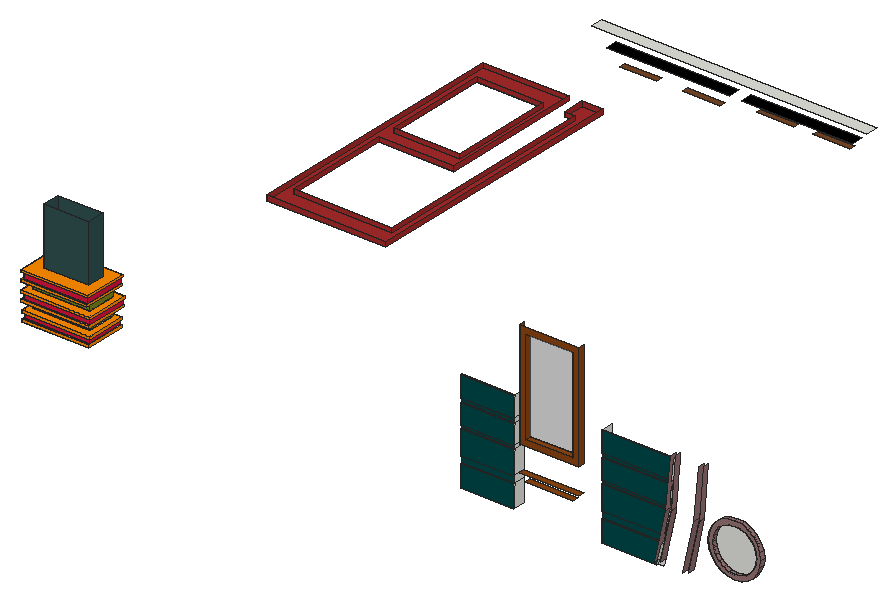
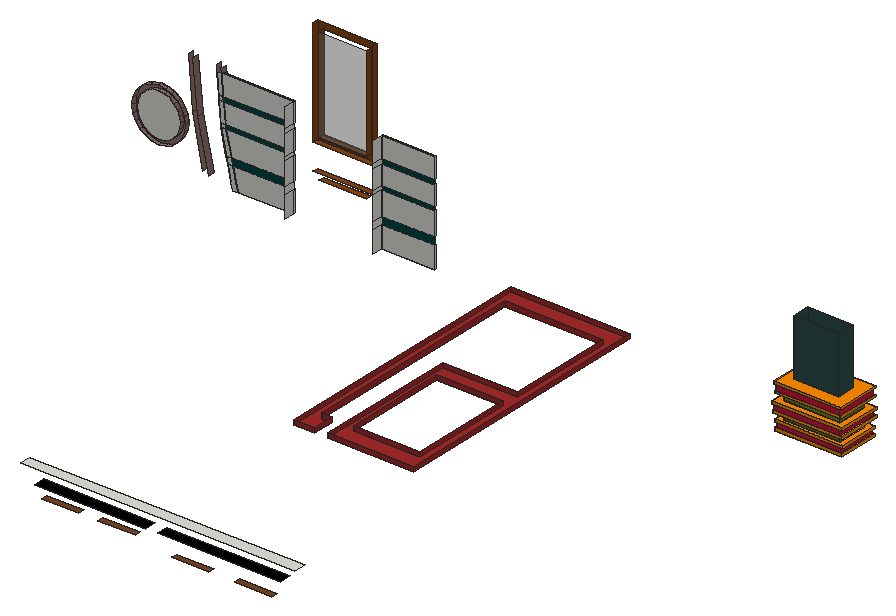
# SketchUp Ruby script. Lengths in inches.
U = 1.inch
M = Sketchup.active_model
def pt(a) = Geom::Point3d.new(a.map { |v| v * U })
def face(e, loops, mat)
  f = e.add_face(loops[0].map { |a| pt(a) })
  loops[1..].each { |l| e.add_face(l.map { |a| pt(a) }).erase! }
  f.material = f.back_material = mat if mat
  f
end
# faces: each face lists its corners as indices into pts; further lists are holes
def faces(e, pts, list, mat = nil) = list.each { |f| face(e, (f[0].is_a?(Array) ? f : [f]).map { |l| l.map { |i| pts[i] } }, mat) }
# xy, xz, yz: faces in a plane at the given z, y or x. An outline is a flat list of corners, or four numbers for a rectangle; further outlines are holes
def ring(l) = l.size == 4 ? [[l[0], l[1]], [l[2], l[1]], [l[2], l[3]], [l[0], l[3]]] : l.each_slice(2).to_a
def flat(e, list, mat, &to3) = list.each { |f| face(e, (f[0].is_a?(Array) ? f : [f]).map { |l| ring(l).map { |u, v| to3.(u, v) } }, mat) }
def xy(e, z, list, mat = nil) = flat(e, list, mat) { |x, y| [x, y, z] }
def xz(e, y, list, mat = nil) = flat(e, list, mat) { |x, z| [x, y, z] }
def yz(e, x, list, mat = nil) = flat(e, list, mat) { |y, z| [x, y, z] }
def lines(e, pts, list) = list.each { |a, b| e.add_line(pt(pts[a]), pt(pts[b])) }
# prism: a flat outline (further loops are holes) pulled along v
def prism(e, loops, v, mat = nil)
  f = face(e, loops, mat); d = Geom::Vector3d.new(v.map { |x| x * U })
  f.pushpull(f.normal.samedirection?(d) ? d.length : -d.length)
end
def box(e, o, s, mat = nil) = prism(e, [[o, [o[0] + s[0], o[1], o[2]], [o[0] + s[0], o[1] + s[1], o[2]], [o[0], o[1] + s[1], o[2]]]], [0, 0, s[2]], mat)
def at(x, y, z, deg = 0) = Geom::Transformation.translation(pt([x, y, z])) * Geom::Transformation.rotation(ORIGIN, Z_AXIS, deg.degrees)
def axes(o, x, y, z) = Geom::Transformation.new([*x, 0, *y, 0, *z, 0, *pt(o).to_a, 1])
def part(name) = M.definitions.add(name)
# library, detail: a bought-in or finely detailed component or shape, given as its bounding box
def library(name, o, s) = part(name).tap { |d| box(d.entities, o, s) }
def detail(e, o, s) = box(e.add_group.entities, o, s)
def put(e, d, t, mat = nil) = e.add_instance(d, t).tap { |i| i.material = mat if mat }
def group(e, t, mat = nil) = e.add_group.tap { |g| g.transformation = t; g.material = mat if mat }.entities
root = M.entities
M.materials.add("[0018_Brown]").color = [165, 42, 42]
M.materials.add("[0019_Crimson]").color = [220, 20, 60]
M.materials.add("[0039_DarkOrange]").color = [255, 140, 0]
M.materials.add("[0043_SaddleBrown]").color = [139, 69, 19]
M.materials.add("[0057_DarkKhaki]").color = [122, 132, 27]
M.materials.add("[0078_DarkSlateGray]").color = [47, 79, 79]
M.materials.add("[0119_RosyBrown]").color = [150, 114, 114]
M.materials.add("[0137_Black]").color = [0, 0, 0]
M.materials.add("[Color H08]").color = [0, 71, 71]
M.materials.add("[Translucent Glass Gray]").color = [128, 128, 128]
M.materials["[Translucent Glass Gray]"].alpha = 0.5
M.materials.add("[Wood Veneer 01]").color = [120, 70, 37]
xy(root,193.52,[[[1.625,647.11,35.57,667.86],[4,651.11,32.57,666.11]]],"[0039_DarkOrange]")
xy(root,194,[[221.0625,650.11,247.97,651.11],[292.45,650.11,320.32,651.11]],"[Color H08]")
xy(root,194.96,[[1.625,647.11,2.4375,648.11]])
xy(root,194.96,[[2.4375,647.11,35.57,647.11,35.57,667.86,1.625,667.86,1.625,648.11,2.4375,648.11,2.4375,667.36,35.13,667.36,35.13,648.11,2.4375,648.11]],"[0039_DarkOrange]")
xy(root,197.25,[[[1.3125,647.11,35.69,667.68],[2.4375,648.11,35.13,667.36]]],"[0039_DarkOrange]")
xy(root,198.71,[[[1.3125,647.11,35.69,667.68],[4,651.11,32.57,666.11]]],"[0039_DarkOrange]")
xy(root,202.27,[[[0.75,647.11,35.57,669.24],[4,651.11,32.57,666.11]]],"[0039_DarkOrange]")
xy(root,203.52,[[[0.75,647.11,35.57,669.24],[1.625,648.11,35.19,668.8]]],"[0039_DarkOrange]")
xy(root,204.94,[[221.0625,650.11,247.97,651.11],[292.45,650.11,323.1,651.11]],"[Color H08]")
xy(root,206.2,[[[0.75,647.11,36,669.24],[1.625,648.11,35.19,668.8]]],"[0039_DarkOrange]")
xy(root,207.46,[[[0.75,647.11,36,669.24],[4,651.11,32.57,666.11]]],"[0039_DarkOrange]")
xy(root,208.59,[[221.0625,650.11,247.97,651.11],[292.45,650.11,323.92,651.11]],"[Color H08]")
xy(root,211.52,[[[1.25,647.11,34.375,669.18],[1.625,648.11,34.13,668.8]]],"[0039_DarkOrange]")
xy(root,211.58,[[[1.625,648.11,34.13,668.8],[4,651.11,32.57,666.11]]],"[0039_DarkOrange]")
xy(root,211.75,[[258.01,645.11,281.88,648.11]],"[0043_SaddleBrown]")
xy(root,212.58,[[1.25,647.11,34.375,647.11,34.375,648.11,1.625,648.11,1.625,668.8,34.13,668.8,34.13,648.11,34.375,648.11,34.375,669.18,1.25,669.18]],"[0039_DarkOrange]")
xy(root,214.75,[[255.01,645.11,284.88,648.11]],"[0043_SaddleBrown]")
xy(root,215.72,[[[0.8125,647.11,34.75,669.36],[1.625,648.11,34.13,668.8]]],"[0039_DarkOrange]")
xy(root,215.75,[[82.37,924.36,101.18,927.36],[114.12,924.36,132.93,927.36]],"[Wood Veneer 01]")
xy(root,216.77,[[7,654.11,29.57,663.11]])
xy(root,216.77,[[[0.8125,647.11,34.75,669.36],[7,654.11,29.57,663.11]]],"[0039_DarkOrange]")
xy(root,219.3125,[[151.49,924.36,170.3,927.36],[179.93,924.36,198.74,927.36]],"[Wood Veneer 01]")
xy(root,220.65,[[221.0625,650.11,247.97,651.11],[292.45,650.11,326.64,651.11]],"[Color H08]")
xy(root,222.41,[[221.0625,650.11,247.97,651.11],[292.45,650.11,326.91,651.11]],"[Color H08]")
xy(root,224.07,[[78.125,921.36,140.28,927.36],[146.28,921.36,202.43,927.36]],"[0137_Black]")
xy(root,227.93,[[255.01,645.11,284.88,648.11]],"[0043_SaddleBrown]")
xy(root,230.93,[[258.01,645.11,281.88,648.11]],"[0043_SaddleBrown]")
xy(root,231.39,[[70.81,921.36,209.75,927.36]])
xy(root,232.54,[[221.0625,650.11,247.97,651.11],[292.45,650.11,327.84,651.11]],"[Color H08]")
xy(root,234.84,[[221.0625,650.11,247.97,651.11],[292.45,650.11,328.05,651.11]],"[Color H08]")
xy(root,243.17,[[[71.2,714.73,71.2,851.92,114.56,851.92,114.56,779.39,76.53,779.39,76.53,725.47,126.31,725.47,126.31,841.18,121.29,841.18,121.29,851.92,131.64,851.92,131.64,714.73],[76.53,788.7,109.94,841.18]]],"[0018_Brown]")
xz(root,645.11,[[[255.01,227.93,284.88,281.93],[258.01,230.93,281.88,278.93]]],"[0043_SaddleBrown]")
xz(root,647.11,[[1.625,193.52,35.57,194.96],[1.3125,197.25,35.69,198.71],[0.75,202.27,35.57,203.52],[0.75,206.2,36,207.46],[1.25,211.52,34.375,212.58],
  [0.8125,215.72,34.75,216.77]],"[0039_DarkOrange]")
xz(root,648.11,[[1.625,211.52,34.13,211.54],[1.625,211.54,34.13,211.58],[1.625,211.58,34.13,212.58]])
xz(root,648.11,[[2.4375,194.96,35.13,197.25],[1.625,203.52,35.19,206.2],[1.625,212.58,34.13,215.72]],"[0019_Crimson]")
xz(root,648.11,[[258.01,230.93,281.88,278.93]],"[Translucent Glass Gray]")
xz(root,649.11,[[[360.63,201.66,364.12,202.12,367.36,203.46,370.15,205.6,372.29,208.39,373.63,211.63,374.09,215.11,373.63,218.6,372.29,221.84,370.15,224.63,367.36,226.76,364.12,228.11,360.63,228.57,357.15,228.11,353.91,226.76,351.12,224.63,348.98,221.84,347.64,218.6,347.18,215.11,347.64,211.63,348.98,208.39,351.12,205.6,353.91,203.46,357.15,202.12],[360.63,204.07,357.78,204.45,355.11,205.55,352.83,207.31,351.07,209.59,349.97,212.26,349.59,215.11,349.97,217.97,351.07,220.64,352.83,222.92,355.11,224.68,357.78,225.78,360.63,226.16,363.49,225.78,366.16,224.68,368.44,222.92,370.2,220.64,371.3,217.97,371.68,215.11,371.3,212.26,370.2,209.59,368.44,207.31,366.16,205.55,363.49,204.45]]],"[0119_RosyBrown]")
xz(root,650.11,[[221.0625,194,247.97,204.94],[292.45,194,320.32,194,321.14,196.24,323.1,204.94,292.45,204.94],[221.0625,208.59,247.97,220.65],[292.45,208.59,323.92,208.59,326.64,220.65,292.45,220.65],[221.0625,222.41,247.97,232.54],
  [292.45,222.41,326.91,222.41,327.84,232.54,292.45,232.54],[221.0625,234.84,247.97,245.03],[292.45,234.84,328.05,234.84,328.99,245.03,292.45,245.03]],"[Color H08]")
xz(root,651.11,[[4,193.52,32.57,198.71],[221.0625,194,247.97,204.94],[292.45,194,292.45,204.94,323.1,204.94,321.14,196.24,320.32,194],[320.32,194,323.04,194,324.26,197.49,325.82,204.94,323.1,204.94,321.14,196.24],[4,202.27,32.57,207.46],
  [360.63,204.07,363.49,204.45,366.16,205.55,368.44,207.31,370.2,209.59,371.3,212.26,371.68,215.11,371.3,217.97,370.2,220.64,368.44,222.92,366.16,224.68,363.49,225.78,360.63,226.16,357.78,225.78,355.11,224.68,352.83,222.92,351.07,220.64,349.97,217.97,349.59,215.11,349.97,212.26,351.07,209.59,352.83,207.31,355.11,205.55,357.78,204.45],[323.1,204.94,325.82,204.94,326.59,208.59,323.92,208.59],[221.0625,208.59,247.97,220.65],[292.45,208.59,292.45,220.65,326.64,220.65,323.92,208.59],[323.92,208.59,326.59,208.59,329.12,220.65,326.64,220.65],
  [326.64,220.65,329.12,220.65,329.49,222.41,326.91,222.41,326.83,221.48],[221.0625,222.41,247.97,232.54],[292.45,222.41,292.45,232.54,327.84,232.54,326.91,222.41],[326.91,222.41,329.49,222.41,329.52,222.56,330.31,232.54,327.84,232.54],[327.84,232.54,330.31,232.54,330.49,234.84,328.05,234.84],
  [221.0625,234.84,247.97,245.03],[292.45,234.84,292.45,245.03,328.99,245.03,328.05,234.84],[328.05,234.84,330.49,234.84,331.29,245.03,328.99,245.03]])
xz(root,651.11,[[4,198.71,32.57,202.27],[4,207.46,32.57,211.58]],"[0057_DarkKhaki]")
xz(root,651.11,[[221.0625,204.94,247.97,208.59],[292.45,204.94,323.1,204.94,323.92,208.59,292.45,208.59],[221.0625,220.65,247.97,222.41],[292.45,220.65,326.64,220.65,326.83,221.48,326.91,222.41,292.45,222.41],[221.0625,232.54,247.97,234.84],
  [292.45,232.54,327.84,232.54,328.05,234.84,292.45,234.84]],"[Color H08]")
xz(root,654.11,[[7,216.77,29.57,245.51]],"[0078_DarkSlateGray]")
xz(root,663.11,[[7,216.77,29.57,245.51]],"[0078_DarkSlateGray]")
xz(root,666.11,[[4,193.52,32.57,198.71],[4,202.27,32.57,207.46]])
xz(root,666.11,[[4,198.71,32.57,202.27],[4,207.46,32.57,211.58]],"[0057_DarkKhaki]")
xz(root,667.36,[[2.4375,194.96,35.13,197.25]],"[0019_Crimson]")
xz(root,667.68,[[1.3125,197.25,35.69,198.71]],"[0039_DarkOrange]")
xz(root,667.86,[[1.625,193.52,35.57,194.96]],"[0039_DarkOrange]")
xz(root,668.8,[[1.625,211.52,34.13,211.58],[1.625,211.58,34.13,212.58]])
xz(root,668.8,[[1.625,203.52,35.19,206.2],[1.625,212.58,34.13,215.72]],"[0019_Crimson]")
xz(root,669.18,[[1.25,211.52,34.375,212.58]],"[0039_DarkOrange]")
xz(root,669.24,[[0.75,202.27,35.57,203.52],[0.75,206.2,36,207.46]],"[0039_DarkOrange]")
xz(root,669.36,[[0.8125,215.72,34.75,216.77]],"[0039_DarkOrange]")
xz(root,714.73,[[71.2,243.17,131.64,245.51]],"[0018_Brown]")
xz(root,725.47,[[76.53,243.17,126.31,245.51]],"[0018_Brown]")
xz(root,779.39,[[76.53,243.17,114.56,245.51]],"[0018_Brown]")
xz(root,788.7,[[76.53,243.17,109.94,245.51]],"[0018_Brown]")
xz(root,841.18,[[76.53,243.17,109.94,245.51],[121.29,243.17,126.31,245.51]],"[0018_Brown]")
xz(root,851.92,[[71.2,243.17,114.56,245.51],[121.29,243.17,131.64,245.51]],"[0018_Brown]")
yz(root,0.75,[[647.11,202.27,669.24,203.52],[647.11,206.2,669.24,207.46]],"[0039_DarkOrange]")
yz(root,0.8125,[[647.11,215.72,669.36,216.77]],"[0039_DarkOrange]")
yz(root,1.25,[[647.11,211.52,669.18,212.58]],"[0039_DarkOrange]")
yz(root,1.3125,[[647.11,197.25,667.68,198.71]],"[0039_DarkOrange]")
yz(root,1.625,[[648.11,211.52,668.8,211.58],[648.11,211.58,668.8,212.58]])
yz(root,1.625,[[648.11,203.52,668.8,206.2],[648.11,212.58,668.8,215.72]],"[0019_Crimson]")
yz(root,1.625,[[647.11,193.52,667.86,194.96]],"[0039_DarkOrange]")
yz(root,2.4375,[[648.11,194.96,667.36,197.25]],"[0019_Crimson]")
yz(root,4,[[651.11,193.52,666.11,198.71],[651.11,202.27,666.11,207.46]])
yz(root,4,[[651.11,198.71,666.11,202.27],[651.11,207.46,666.11,211.58]],"[0057_DarkKhaki]")
yz(root,7,[[654.11,216.77,663.11,245.51]],"[0078_DarkSlateGray]")
yz(root,29.57,[[654.11,216.77,663.11,245.51]],"[0078_DarkSlateGray]")
yz(root,32.57,[[651.11,193.52,666.11,198.71],[651.11,202.27,666.11,207.46]])
yz(root,32.57,[[651.11,198.71,666.11,202.27],[651.11,207.46,666.11,211.58]],"[0057_DarkKhaki]")
yz(root,34.13,[[648.11,211.52,668.8,211.58],[648.11,211.58,668.8,212.58]])
yz(root,34.13,[[648.11,212.58,668.8,215.72]],"[0019_Crimson]")
yz(root,34.375,[[647.11,211.52,669.18,212.58]],"[0039_DarkOrange]")
yz(root,34.75,[[647.11,215.72,669.36,216.77]],"[0039_DarkOrange]")
yz(root,35.13,[[648.11,193.52,667.36,194.96]])
yz(root,35.13,[[648.11,194.96,667.36,197.25]],"[0019_Crimson]")
yz(root,35.19,[[648.11,203.52,668.8,206.2]],"[0019_Crimson]")
yz(root,35.57,[[647.11,193.52,667.86,194.96],[647.11,202.27,669.24,203.52]],"[0039_DarkOrange]")
yz(root,35.69,[[647.11,197.25,667.68,198.71]],"[0039_DarkOrange]")
yz(root,36,[[647.11,206.2,669.24,207.46]],"[0039_DarkOrange]")
yz(root,71.2,[[714.73,243.17,851.92,245.51]],"[0018_Brown]")
yz(root,76.53,[[725.47,243.17,779.39,245.51],[788.7,243.17,841.18,245.51]],"[0018_Brown]")
yz(root,109.94,[[788.7,243.17,841.18,245.51]],"[0018_Brown]")
yz(root,114.56,[[779.39,243.17,851.92,245.51]],"[0018_Brown]")
yz(root,121.29,[[841.18,243.17,851.92,245.51]],"[0018_Brown]")
yz(root,126.31,[[725.47,243.17,841.18,245.51]],"[0018_Brown]")
yz(root,131.64,[[714.73,243.17,851.92,245.51]],"[0018_Brown]")
yz(root,221.0625,[[650.11,194,651.11,204.94],[650.11,208.59,651.11,220.65],[650.11,222.41,651.11,232.54],[650.11,234.84,651.11,245.03]])
yz(root,247.97,[[650.11,194,651.11,204.94],[651.11,194,656.36,204.94],[651.11,204.94,656.36,208.59],[650.11,208.59,651.11,220.65],[651.11,208.59,656.36,220.65],
  [651.11,220.65,656.36,222.41],[650.11,222.41,651.11,232.54],[651.11,222.41,656.36,232.54],[651.11,232.54,656.36,234.84],[650.11,234.84,651.11,245.03],
  [651.11,234.84,656.36,245.03]])
yz(root,255.01,[[645.11,227.93,648.11,281.93]],"[0043_SaddleBrown]")
yz(root,258.01,[[645.11,230.93,648.11,278.93]],"[0043_SaddleBrown]")
yz(root,281.88,[[645.11,230.93,648.11,278.93]],"[0043_SaddleBrown]")
yz(root,284.88,[[645.11,227.93,648.11,281.93]],"[0043_SaddleBrown]")
yz(root,292.45,[[650.11,194,651.11,204.94],[651.11,194,656.36,204.94],[651.11,204.94,656.36,208.59],[650.11,208.59,651.11,220.65],[651.11,208.59,656.36,220.65],
  [651.11,220.65,656.36,222.41],[650.11,222.41,651.11,232.54],[651.11,222.41,656.36,232.54],[651.11,232.54,656.36,234.84],[650.11,234.84,651.11,245.03],
  [651.11,234.84,656.36,245.03]])
p = [[321.14,651.11,196.24],[320.32,651.11,194],[320.32,650.11,194],[321.14,650.11,196.24],[323.92,651.11,208.59],[323.1,651.11,204.94],
  [323.1,650.11,204.94],[321.14,648.11,196.24],[326.83,648.11,221.48],[326.83,651.11,221.48],[326.64,651.11,220.65],[326.64,650.11,220.65],
  [323.92,650.11,208.59],[340.9,651.11,221.48],[335.22,651.11,196.24],[335.22,648.11,196.24],[340.9,648.11,221.48],[324.26,651.11,197.49],
  [325.82,651.11,204.94],[326.59,651.11,208.59],[329.12,651.11,220.65],[329.49,651.11,222.41],[329.52,651.11,222.56],[329.52,648.11,222.56],
  [324.26,648.11,197.49],[338.33,651.11,197.49],[343.6,651.11,222.56],[343.6,648.11,222.56],[338.33,648.11,197.49],[357.15,651.11,202.12],
  [360.63,651.11,201.66],[360.63,649.11,201.66],[357.15,649.11,202.12],[364.12,651.11,202.12],[364.12,649.11,202.12],[353.91,651.11,203.46],
  [353.91,649.11,203.46],[367.36,651.11,203.46],[367.36,649.11,203.46],[351.12,651.11,205.6],[351.12,649.11,205.6],[370.15,651.11,205.6],
  [370.15,649.11,205.6],[360.63,651.11,204.07],[357.78,651.11,204.45],[357.78,649.11,204.45],[360.63,649.11,204.07],[363.49,651.11,204.45],
  [363.49,649.11,204.45],[355.11,651.11,205.55],[355.11,649.11,205.55],[366.16,651.11,205.55],[366.16,649.11,205.55],[348.98,651.11,208.39],
  [348.98,649.11,208.39],[352.83,651.11,207.31],[352.83,649.11,207.31],[368.44,651.11,207.31],[368.44,649.11,207.31],[372.29,651.11,208.39],
  [372.29,649.11,208.39],[351.07,651.11,209.59],[351.07,649.11,209.59],[370.2,651.11,209.59],[370.2,649.11,209.59],[347.64,651.11,211.63],
  [347.64,649.11,211.63],[373.63,651.11,211.63],[373.63,649.11,211.63],[349.97,651.11,212.26],[349.97,649.11,212.26],[371.3,651.11,212.26],
  [371.3,649.11,212.26],[347.18,651.11,215.11],[347.18,649.11,215.11],[374.09,651.11,215.11],[374.09,649.11,215.11],[349.59,651.11,215.11],
  [349.59,649.11,215.11],[371.68,651.11,215.11],[371.68,649.11,215.11],[347.64,651.11,218.6],[347.64,649.11,218.6],[349.97,651.11,217.97],
  [349.97,649.11,217.97],[371.3,651.11,217.97],[371.3,649.11,217.97],[373.63,651.11,218.6],[373.63,649.11,218.6],[351.07,651.11,220.64],
  [351.07,649.11,220.64],[370.2,651.11,220.64],[370.2,649.11,220.64],[348.98,651.11,221.84],[348.98,649.11,221.84],[372.29,651.11,221.84],
  [372.29,649.11,221.84],[352.83,651.11,222.92],[352.83,649.11,222.92],[368.44,651.11,222.92],[368.44,649.11,222.92],[326.91,651.11,222.41],
  [329.19,648.11,247.23],[329.19,651.11,247.23],[328.99,651.11,245.03],[328.99,650.11,245.03],[328.05,650.11,234.84],[328.05,651.11,234.84],
  [327.84,651.11,232.54],[327.84,650.11,232.54],[326.91,650.11,222.41],[343.27,651.11,247.23],[343.27,648.11,247.23],[351.12,651.11,224.63],
  [351.12,649.11,224.63],[370.15,651.11,224.63],[370.15,649.11,224.63],[330.31,651.11,232.54],[330.49,651.11,234.84],[331.29,651.11,245.03],
  [331.5,651.11,247.73],[331.53,651.11,248.09],[331.53,648.11,248.09],[345.61,651.11,248.09],[345.61,648.11,248.09],[355.11,651.11,224.68],
  [355.11,649.11,224.68],[366.16,651.11,224.68],[366.16,649.11,224.68],[353.91,651.11,226.76],[353.91,649.11,226.76],[367.36,651.11,226.76],
  [367.36,649.11,226.76],[357.78,651.11,225.78],[357.78,649.11,225.78],[363.49,651.11,225.78],[363.49,649.11,225.78],[360.63,651.11,226.16],
  [360.63,649.11,226.16],[357.15,651.11,228.11],[357.15,649.11,228.11],[364.12,651.11,228.11],[364.12,649.11,228.11],[360.63,651.11,228.57],
  [360.63,649.11,228.57],[34.13,668.8,216.77],[34.13,668.8,215.72],[35.19,648.11,207.46],[35.19,648.11,206.2],[35.19,668.8,207.46],
  [35.19,668.8,206.2],[1.625,668.8,207.46],[1.625,668.8,206.2],[1.625,648.11,202.27],[1.625,648.11,203.52],[35.13,648.11,198.71],
  [35.13,648.11,197.25],[35.13,667.36,198.71],[35.13,667.36,197.25],[35.19,648.11,203.52],[35.19,648.11,202.27],[2.4375,648.11,197.25],
  [2.4375,648.11,198.71],[35.13,648.11,193.52],[35.13,648.11,193.5],[34.13,648.11,211.58],[34.13,647.11,211.58],[1.625,668.8,203.52],
  [1.625,668.8,202.27],[2.4375,667.36,197.25],[2.4375,667.36,198.71],[35.19,668.8,203.52],[35.19,668.8,202.27],[35.19,669.24,207.46],
  [34.13,648.11,216.77],[34.13,648.11,215.72]]
faces(root,p,[[0,1,2,3],[5,0,3,6],[10,4,12,11],[108,101,110,109],[104,107,106,105]])
faces(root,p,[[4,5,6,3,7,8,9,10,11,12],[13,14,15,16],[17,18,19,20,21,22,23,24],[25,26,27,28],[29,30,31,32],[30,33,34,31],[35,29,32,36],[33,37,38,34],
  [39,35,36,40],[37,41,42,38],[43,44,45,46],[47,43,46,48],[44,49,50,45],[51,47,48,52],[53,39,40,54],[49,55,56,50],
  [57,51,52,58],[41,59,60,42],[55,61,62,56],[63,57,58,64],[65,53,54,66],[59,67,68,60],[61,69,70,62],[71,63,64,72],
  [73,65,66,74],[67,75,76,68],[69,77,78,70],[79,71,72,80],[81,73,74,82],[77,83,84,78],[85,79,80,86],[75,87,88,76],
  [83,89,90,84],[91,85,86,92],[93,81,82,94],[87,95,96,88],[89,97,98,90],[99,91,92,100],[101,9,8,102,103,104,105,106,107,108,109,110],[111,13,16,112],
  [113,93,94,114],[95,115,116,96],[22,117,118,119,120,121,122,23],[26,123,124,27],[97,125,126,98],[127,99,100,128],[129,113,114,130],[115,131,132,116],
  [125,133,134,126],[135,127,128,136],[133,137,138,134],[137,135,136,138],[139,129,130,140],[131,141,142,132],[143,139,140,144],[141,143,144,142]],"[0119_RosyBrown]")
lines(root,p,[[145,146],[147,148],[149,150],[151,152],[153,154],[155,156],[157,158],[159,160],[161,162],[163,164],[165,166],[167,168],
  [169,170],[171,172],[149,173],[174,175]])
